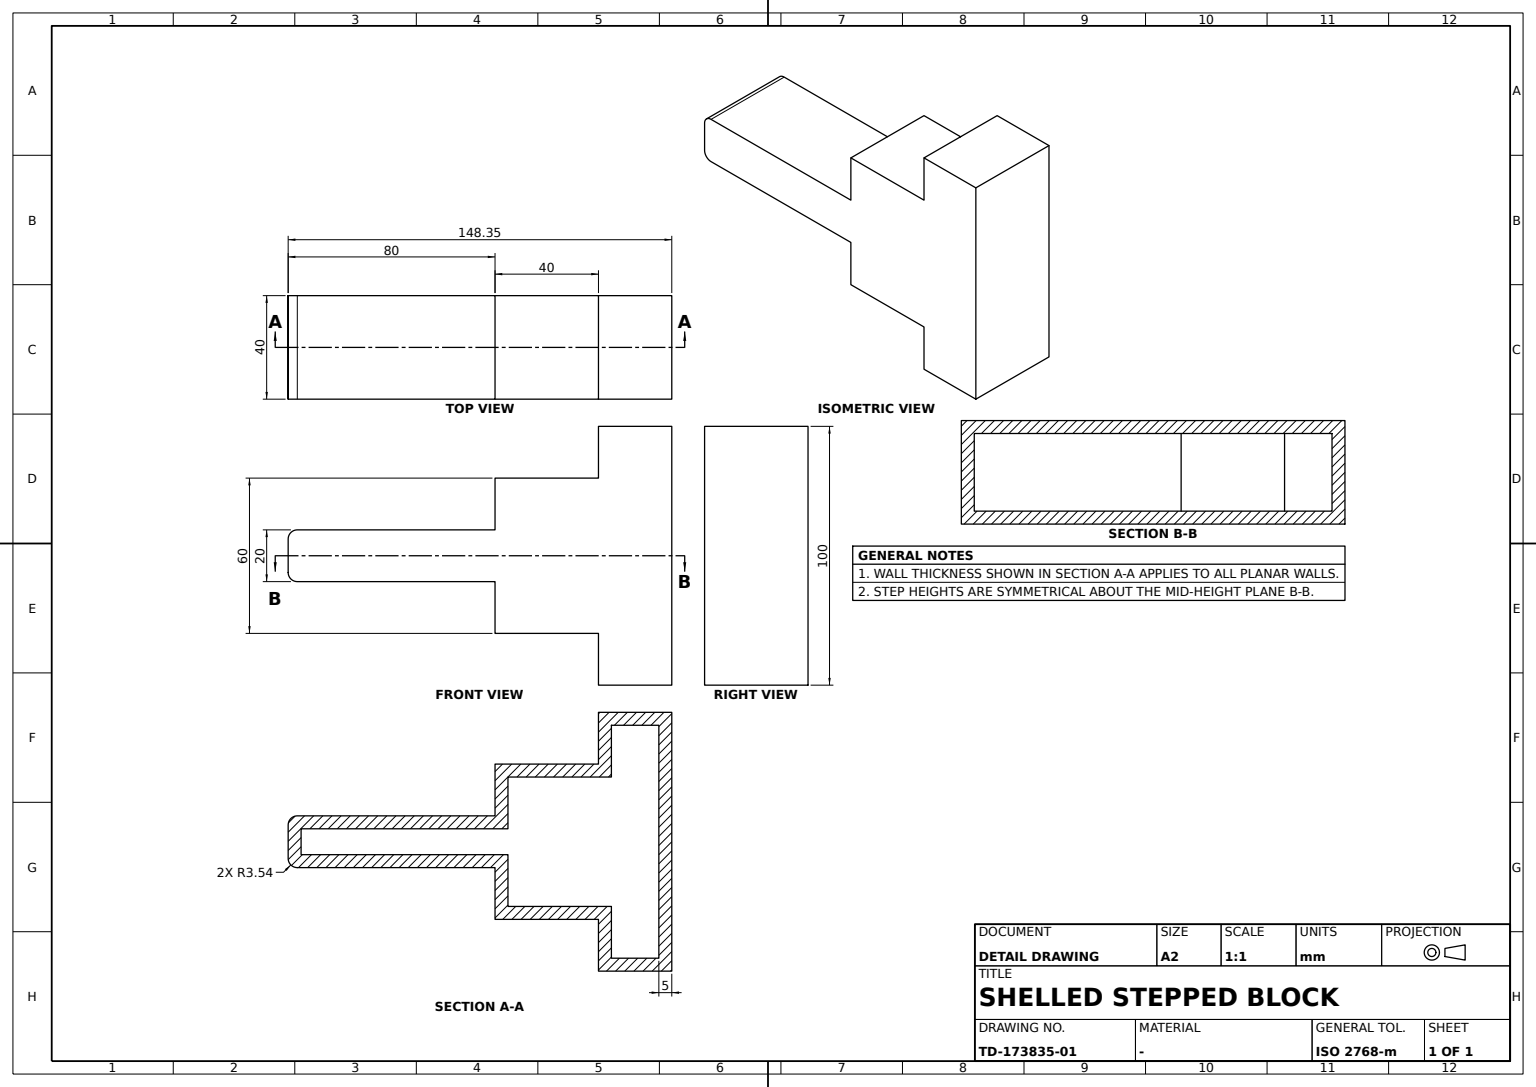
ISO-10303-21;
HEADER;
FILE_DESCRIPTION((''),'2;1');
FILE_NAME('','',(''),(''),'','','');
FILE_SCHEMA(('AUTOMOTIVE_DESIGN'));
ENDSEC;
DATA;
#1=APPLICATION_CONTEXT('');
#2=PRODUCT_CONTEXT('',#1,'mechanical');
#3=PRODUCT('','','',(#2));
#4=PRODUCT_DEFINITION_FORMATION('','',#3);
#5=PRODUCT_DEFINITION_CONTEXT('',#1,'design');
#6=PRODUCT_DEFINITION('','',#4,#5);
#7=PRODUCT_DEFINITION_SHAPE('','',#6);
#8=(LENGTH_UNIT()NAMED_UNIT(*)SI_UNIT(.MILLI.,.METRE.));
#9=(NAMED_UNIT(*)PLANE_ANGLE_UNIT()SI_UNIT($,.RADIAN.));
#10=(NAMED_UNIT(*)SI_UNIT($,.STERADIAN.)SOLID_ANGLE_UNIT());
#11=UNCERTAINTY_MEASURE_WITH_UNIT(LENGTH_MEASURE(0.005),#8,'distance_accuracy_value','');
#12=(GEOMETRIC_REPRESENTATION_CONTEXT(3)GLOBAL_UNCERTAINTY_ASSIGNED_CONTEXT((#11))GLOBAL_UNIT_ASSIGNED_CONTEXT((#8,#9,#10))REPRESENTATION_CONTEXT('',''));
#13=CARTESIAN_POINT('',(-28.352545,30.,-20.));
#14=VERTEX_POINT('',#13);
#15=CARTESIAN_POINT('',(-28.352545,30.,20.));
#16=VERTEX_POINT('',#15);
#17=CARTESIAN_POINT('',(-28.352545,30.,0.));
#18=DIRECTION('',(0.,0.,1.));
#19=VECTOR('',#18,1000.);
#20=LINE('',#17,#19);
#21=EDGE_CURVE('',#14,#16,#20,.T.);
#22=ORIENTED_EDGE('',*,*,#21,.F.);
#23=CARTESIAN_POINT('',(-68.352545,30.,-20.));
#24=VERTEX_POINT('',#23);
#25=CARTESIAN_POINT('',(0.,30.,-20.));
#26=DIRECTION('',(-1.,0.,0.));
#27=VECTOR('',#26,1000.);
#28=LINE('',#25,#27);
#29=EDGE_CURVE('',#14,#24,#28,.T.);
#30=ORIENTED_EDGE('',*,*,#29,.T.);
#31=CARTESIAN_POINT('',(-68.352545,30.,20.));
#32=VERTEX_POINT('',#31);
#33=CARTESIAN_POINT('',(-68.352545,30.,0.));
#34=LINE('',#33,#19);
#35=EDGE_CURVE('',#24,#32,#34,.T.);
#36=ORIENTED_EDGE('',*,*,#35,.T.);
#37=CARTESIAN_POINT('',(0.,30.,20.));
#38=LINE('',#37,#27);
#39=EDGE_CURVE('',#16,#32,#38,.T.);
#40=ORIENTED_EDGE('',*,*,#39,.F.);
#41=EDGE_LOOP('',(#22,#30,#36,#40));
#42=FACE_BOUND('',#41,.T.);
#43=DIRECTION('',(0.,1.,0.));
#44=AXIS2_PLACEMENT_3D('',#17,#43,#26);
#45=PLANE('',#44);
#46=ADVANCED_FACE('',(#42),#45,.T.);
#47=CARTESIAN_POINT('',(-68.352545,10.,-20.));
#48=VERTEX_POINT('',#47);
#49=CARTESIAN_POINT('',(-68.352545,10.,20.));
#50=VERTEX_POINT('',#49);
#51=CARTESIAN_POINT('',(-68.352545,10.,0.));
#52=LINE('',#51,#19);
#53=EDGE_CURVE('',#48,#50,#52,.T.);
#54=ORIENTED_EDGE('',*,*,#53,.T.);
#55=CARTESIAN_POINT('',(-68.352545,0.,20.));
#56=DIRECTION('',(0.,-1.,0.));
#57=VECTOR('',#56,1000.);
#58=LINE('',#55,#57);
#59=EDGE_CURVE('',#32,#50,#58,.T.);
#60=ORIENTED_EDGE('',*,*,#59,.F.);
#61=ORIENTED_EDGE('',*,*,#35,.F.);
#62=CARTESIAN_POINT('',(-68.352545,0.,-20.));
#63=LINE('',#62,#57);
#64=EDGE_CURVE('',#24,#48,#63,.T.);
#65=ORIENTED_EDGE('',*,*,#64,.T.);
#66=EDGE_LOOP('',(#54,#60,#61,#65));
#67=FACE_BOUND('',#66,.T.);
#68=AXIS2_PLACEMENT_3D('',#33,#26,#56);
#69=PLANE('',#68);
#70=ADVANCED_FACE('',(#67),#69,.T.);
#71=CARTESIAN_POINT('',(-28.352545,-30.,-20.));
#72=VERTEX_POINT('',#71);
#73=CARTESIAN_POINT('',(-28.352545,-30.,20.));
#74=VERTEX_POINT('',#73);
#75=CARTESIAN_POINT('',(-28.352545,-30.,0.));
#76=LINE('',#75,#19);
#77=EDGE_CURVE('',#72,#74,#76,.T.);
#78=ORIENTED_EDGE('',*,*,#77,.T.);
#79=CARTESIAN_POINT('',(-68.352545,-30.,20.));
#80=VERTEX_POINT('',#79);
#81=CARTESIAN_POINT('',(0.,-30.,20.));
#82=DIRECTION('',(1.,0.,0.));
#83=VECTOR('',#82,1000.);
#84=LINE('',#81,#83);
#85=EDGE_CURVE('',#80,#74,#84,.T.);
#86=ORIENTED_EDGE('',*,*,#85,.F.);
#87=CARTESIAN_POINT('',(-68.352545,-30.,-20.));
#88=VERTEX_POINT('',#87);
#89=CARTESIAN_POINT('',(-68.352545,-30.,0.));
#90=LINE('',#89,#19);
#91=EDGE_CURVE('',#88,#80,#90,.T.);
#92=ORIENTED_EDGE('',*,*,#91,.F.);
#93=CARTESIAN_POINT('',(0.,-30.,-20.));
#94=LINE('',#93,#83);
#95=EDGE_CURVE('',#88,#72,#94,.T.);
#96=ORIENTED_EDGE('',*,*,#95,.T.);
#97=EDGE_LOOP('',(#78,#86,#92,#96));
#98=FACE_BOUND('',#97,.T.);
#99=AXIS2_PLACEMENT_3D('',#89,#56,#82);
#100=PLANE('',#99);
#101=ADVANCED_FACE('',(#98),#100,.T.);
#102=CARTESIAN_POINT('',(0.,-50.,20.));
#103=VERTEX_POINT('',#102);
#104=CARTESIAN_POINT('',(-28.352545,-50.,20.));
#105=VERTEX_POINT('',#104);
#106=LINE('',#102,#27);
#107=EDGE_CURVE('',#103,#105,#106,.T.);
#108=ORIENTED_EDGE('',*,*,#107,.F.);
#109=CARTESIAN_POINT('',(0.,50.,20.));
#110=VERTEX_POINT('',#109);
#111=CARTESIAN_POINT('',(0.,0.,20.));
#112=VECTOR('',#43,1000.);
#113=LINE('',#111,#112);
#114=EDGE_CURVE('',#103,#110,#113,.T.);
#115=ORIENTED_EDGE('',*,*,#114,.T.);
#116=CARTESIAN_POINT('',(-28.352545,50.,20.));
#117=VERTEX_POINT('',#116);
#118=LINE('',#109,#27);
#119=EDGE_CURVE('',#110,#117,#118,.T.);
#120=ORIENTED_EDGE('',*,*,#119,.T.);
#121=CARTESIAN_POINT('',(-28.352545,0.,20.));
#122=LINE('',#121,#57);
#123=EDGE_CURVE('',#117,#16,#122,.T.);
#124=ORIENTED_EDGE('',*,*,#123,.T.);
#125=ORIENTED_EDGE('',*,*,#39,.T.);
#126=ORIENTED_EDGE('',*,*,#59,.T.);
#127=CARTESIAN_POINT('',(-144.817011,10.,20.));
#128=VERTEX_POINT('',#127);
#129=CARTESIAN_POINT('',(0.,10.,20.));
#130=LINE('',#129,#27);
#131=EDGE_CURVE('',#50,#128,#130,.T.);
#132=ORIENTED_EDGE('',*,*,#131,.T.);
#133=CARTESIAN_POINT('',(-148.352545,6.464466,20.));
#134=VERTEX_POINT('',#133);
#135=CARTESIAN_POINT('',(-144.817011,6.464466,20.));
#136=AXIS2_PLACEMENT_3D('',#135,#18,#82);
#137=CIRCLE('',#136,3.535534);
#138=EDGE_CURVE('',#128,#134,#137,.T.);
#139=ORIENTED_EDGE('',*,*,#138,.T.);
#140=CARTESIAN_POINT('',(-148.352545,-6.464466,20.));
#141=VERTEX_POINT('',#140);
#142=CARTESIAN_POINT('',(-148.352545,0.,20.));
#143=LINE('',#142,#57);
#144=EDGE_CURVE('',#134,#141,#143,.T.);
#145=ORIENTED_EDGE('',*,*,#144,.T.);
#146=CARTESIAN_POINT('',(-144.817011,-10.,20.));
#147=VERTEX_POINT('',#146);
#148=CARTESIAN_POINT('',(-144.817011,-6.464466,20.));
#149=AXIS2_PLACEMENT_3D('',#148,#18,#82);
#150=CIRCLE('',#149,3.535534);
#151=EDGE_CURVE('',#141,#147,#150,.T.);
#152=ORIENTED_EDGE('',*,*,#151,.T.);
#153=CARTESIAN_POINT('',(-68.352545,-10.,20.));
#154=VERTEX_POINT('',#153);
#155=CARTESIAN_POINT('',(0.,-10.,20.));
#156=LINE('',#155,#83);
#157=EDGE_CURVE('',#147,#154,#156,.T.);
#158=ORIENTED_EDGE('',*,*,#157,.T.);
#159=EDGE_CURVE('',#154,#80,#58,.T.);
#160=ORIENTED_EDGE('',*,*,#159,.T.);
#161=ORIENTED_EDGE('',*,*,#85,.T.);
#162=EDGE_CURVE('',#74,#105,#122,.T.);
#163=ORIENTED_EDGE('',*,*,#162,.T.);
#164=EDGE_LOOP('',(#108,#115,#120,#124,#125,#126,#132,#139,#145,#152,#158,#160,#161,#163));
#165=FACE_BOUND('',#164,.T.);
#166=AXIS2_PLACEMENT_3D('',#111,#18,#82);
#167=PLANE('',#166);
#168=ADVANCED_FACE('',(#165),#167,.T.);
#169=CARTESIAN_POINT('',(-28.352545,-50.,-20.));
#170=VERTEX_POINT('',#169);
#171=CARTESIAN_POINT('',(-28.352545,0.,-20.));
#172=LINE('',#171,#57);
#173=EDGE_CURVE('',#72,#170,#172,.T.);
#174=ORIENTED_EDGE('',*,*,#173,.T.);
#175=CARTESIAN_POINT('',(-28.352545,-50.,0.));
#176=LINE('',#175,#19);
#177=EDGE_CURVE('',#170,#105,#176,.T.);
#178=ORIENTED_EDGE('',*,*,#177,.T.);
#179=ORIENTED_EDGE('',*,*,#162,.F.);
#180=ORIENTED_EDGE('',*,*,#77,.F.);
#181=EDGE_LOOP('',(#174,#178,#179,#180));
#182=FACE_BOUND('',#181,.T.);
#183=CARTESIAN_POINT('',(-28.352545,50.,0.));
#184=AXIS2_PLACEMENT_3D('',#183,#26,#56);
#185=PLANE('',#184);
#186=ADVANCED_FACE('',(#182),#185,.T.);
#187=ORIENTED_EDGE('',*,*,#29,.F.);
#188=CARTESIAN_POINT('',(-28.352545,50.,-20.));
#189=VERTEX_POINT('',#188);
#190=EDGE_CURVE('',#189,#14,#172,.T.);
#191=ORIENTED_EDGE('',*,*,#190,.F.);
#192=CARTESIAN_POINT('',(0.,50.,-20.));
#193=VERTEX_POINT('',#192);
#194=LINE('',#192,#27);
#195=EDGE_CURVE('',#193,#189,#194,.T.);
#196=ORIENTED_EDGE('',*,*,#195,.F.);
#197=CARTESIAN_POINT('',(0.,-50.,-20.));
#198=VERTEX_POINT('',#197);
#199=CARTESIAN_POINT('',(0.,0.,-20.));
#200=LINE('',#199,#112);
#201=EDGE_CURVE('',#198,#193,#200,.T.);
#202=ORIENTED_EDGE('',*,*,#201,.F.);
#203=LINE('',#197,#27);
#204=EDGE_CURVE('',#198,#170,#203,.T.);
#205=ORIENTED_EDGE('',*,*,#204,.T.);
#206=ORIENTED_EDGE('',*,*,#173,.F.);
#207=ORIENTED_EDGE('',*,*,#95,.F.);
#208=CARTESIAN_POINT('',(-68.352545,-10.,-20.));
#209=VERTEX_POINT('',#208);
#210=EDGE_CURVE('',#209,#88,#63,.T.);
#211=ORIENTED_EDGE('',*,*,#210,.F.);
#212=CARTESIAN_POINT('',(-144.817011,-10.,-20.));
#213=VERTEX_POINT('',#212);
#214=CARTESIAN_POINT('',(0.,-10.,-20.));
#215=LINE('',#214,#83);
#216=EDGE_CURVE('',#213,#209,#215,.T.);
#217=ORIENTED_EDGE('',*,*,#216,.F.);
#218=CARTESIAN_POINT('',(-148.352545,-6.464466,-20.));
#219=VERTEX_POINT('',#218);
#220=CARTESIAN_POINT('',(-144.817011,-6.464466,-20.));
#221=AXIS2_PLACEMENT_3D('',#220,#18,#82);
#222=CIRCLE('',#221,3.535534);
#223=EDGE_CURVE('',#219,#213,#222,.T.);
#224=ORIENTED_EDGE('',*,*,#223,.F.);
#225=CARTESIAN_POINT('',(-148.352545,6.464466,-20.));
#226=VERTEX_POINT('',#225);
#227=CARTESIAN_POINT('',(-148.352545,0.,-20.));
#228=LINE('',#227,#57);
#229=EDGE_CURVE('',#226,#219,#228,.T.);
#230=ORIENTED_EDGE('',*,*,#229,.F.);
#231=CARTESIAN_POINT('',(-144.817011,10.,-20.));
#232=VERTEX_POINT('',#231);
#233=CARTESIAN_POINT('',(-144.817011,6.464466,-20.));
#234=AXIS2_PLACEMENT_3D('',#233,#18,#82);
#235=CIRCLE('',#234,3.535534);
#236=EDGE_CURVE('',#232,#226,#235,.T.);
#237=ORIENTED_EDGE('',*,*,#236,.F.);
#238=CARTESIAN_POINT('',(0.,10.,-20.));
#239=LINE('',#238,#27);
#240=EDGE_CURVE('',#48,#232,#239,.T.);
#241=ORIENTED_EDGE('',*,*,#240,.F.);
#242=ORIENTED_EDGE('',*,*,#64,.F.);
#243=EDGE_LOOP('',(#187,#191,#196,#202,#205,#206,#207,#211,#217,#224,#230,#237,#241,#242));
#244=FACE_BOUND('',#243,.T.);
#245=AXIS2_PLACEMENT_3D('',#199,#18,#82);
#246=PLANE('',#245);
#247=ADVANCED_FACE('',(#244),#246,.F.);
#248=ORIENTED_EDGE('',*,*,#144,.F.);
#249=CARTESIAN_POINT('',(-148.352545,6.464466,0.));
#250=DIRECTION('',(0.,0.,-1.));
#251=VECTOR('',#250,1000.);
#252=LINE('',#249,#251);
#253=EDGE_CURVE('',#134,#226,#252,.T.);
#254=ORIENTED_EDGE('',*,*,#253,.T.);
#255=ORIENTED_EDGE('',*,*,#229,.T.);
#256=CARTESIAN_POINT('',(-148.352545,-6.464466,0.));
#257=LINE('',#256,#251);
#258=EDGE_CURVE('',#141,#219,#257,.T.);
#259=ORIENTED_EDGE('',*,*,#258,.F.);
#260=EDGE_LOOP('',(#248,#254,#255,#259));
#261=FACE_BOUND('',#260,.T.);
#262=CARTESIAN_POINT('',(-148.352545,10.,0.));
#263=AXIS2_PLACEMENT_3D('',#262,#26,#56);
#264=PLANE('',#263);
#265=ADVANCED_FACE('',(#261),#264,.T.);
#266=ORIENTED_EDGE('',*,*,#151,.F.);
#267=ORIENTED_EDGE('',*,*,#258,.T.);
#268=ORIENTED_EDGE('',*,*,#223,.T.);
#269=CARTESIAN_POINT('',(-144.817011,-10.,0.));
#270=LINE('',#269,#251);
#271=EDGE_CURVE('',#147,#213,#270,.T.);
#272=ORIENTED_EDGE('',*,*,#271,.F.);
#273=EDGE_LOOP('',(#266,#267,#268,#272));
#274=FACE_BOUND('',#273,.T.);
#275=CARTESIAN_POINT('',(-144.817011,-6.464466,0.));
#276=AXIS2_PLACEMENT_3D('',#275,#250,#56);
#277=CYLINDRICAL_SURFACE('',#276,3.535534);
#278=ADVANCED_FACE('',(#274),#277,.T.);
#279=LINE('',#183,#19);
#280=EDGE_CURVE('',#189,#117,#279,.T.);
#281=ORIENTED_EDGE('',*,*,#280,.F.);
#282=ORIENTED_EDGE('',*,*,#190,.T.);
#283=ORIENTED_EDGE('',*,*,#21,.T.);
#284=ORIENTED_EDGE('',*,*,#123,.F.);
#285=EDGE_LOOP('',(#281,#282,#283,#284));
#286=FACE_BOUND('',#285,.T.);
#287=ADVANCED_FACE('',(#286),#185,.T.);
#288=ORIENTED_EDGE('',*,*,#107,.T.);
#289=ORIENTED_EDGE('',*,*,#177,.F.);
#290=ORIENTED_EDGE('',*,*,#204,.F.);
#291=CARTESIAN_POINT('',(0.,-50.,0.));
#292=LINE('',#291,#19);
#293=EDGE_CURVE('',#198,#103,#292,.T.);
#294=ORIENTED_EDGE('',*,*,#293,.T.);
#295=EDGE_LOOP('',(#288,#289,#290,#294));
#296=FACE_BOUND('',#295,.T.);
#297=AXIS2_PLACEMENT_3D('',#291,#43,#26);
#298=PLANE('',#297);
#299=ADVANCED_FACE('',(#296),#298,.F.);
#300=ORIENTED_EDGE('',*,*,#53,.F.);
#301=ORIENTED_EDGE('',*,*,#240,.T.);
#302=CARTESIAN_POINT('',(-144.817011,10.,0.));
#303=LINE('',#302,#251);
#304=EDGE_CURVE('',#128,#232,#303,.T.);
#305=ORIENTED_EDGE('',*,*,#304,.F.);
#306=ORIENTED_EDGE('',*,*,#131,.F.);
#307=EDGE_LOOP('',(#300,#301,#305,#306));
#308=FACE_BOUND('',#307,.T.);
#309=AXIS2_PLACEMENT_3D('',#51,#43,#26);
#310=PLANE('',#309);
#311=ADVANCED_FACE('',(#308),#310,.T.);
#312=CARTESIAN_POINT('',(0.,50.,0.));
#313=LINE('',#312,#19);
#314=EDGE_CURVE('',#193,#110,#313,.T.);
#315=ORIENTED_EDGE('',*,*,#314,.F.);
#316=ORIENTED_EDGE('',*,*,#195,.T.);
#317=ORIENTED_EDGE('',*,*,#280,.T.);
#318=ORIENTED_EDGE('',*,*,#119,.F.);
#319=EDGE_LOOP('',(#315,#316,#317,#318));
#320=FACE_BOUND('',#319,.T.);
#321=AXIS2_PLACEMENT_3D('',#312,#43,#26);
#322=PLANE('',#321);
#323=ADVANCED_FACE('',(#320),#322,.T.);
#324=ORIENTED_EDGE('',*,*,#159,.F.);
#325=CARTESIAN_POINT('',(-68.352545,-10.,0.));
#326=LINE('',#325,#19);
#327=EDGE_CURVE('',#209,#154,#326,.T.);
#328=ORIENTED_EDGE('',*,*,#327,.F.);
#329=ORIENTED_EDGE('',*,*,#210,.T.);
#330=ORIENTED_EDGE('',*,*,#91,.T.);
#331=EDGE_LOOP('',(#324,#328,#329,#330));
#332=FACE_BOUND('',#331,.T.);
#333=ADVANCED_FACE('',(#332),#69,.T.);
#334=ORIENTED_EDGE('',*,*,#236,.T.);
#335=ORIENTED_EDGE('',*,*,#253,.F.);
#336=ORIENTED_EDGE('',*,*,#138,.F.);
#337=ORIENTED_EDGE('',*,*,#304,.T.);
#338=EDGE_LOOP('',(#334,#335,#336,#337));
#339=FACE_BOUND('',#338,.T.);
#340=CARTESIAN_POINT('',(-144.817011,6.464466,0.));
#341=AXIS2_PLACEMENT_3D('',#340,#250,#26);
#342=CYLINDRICAL_SURFACE('',#341,3.535534);
#343=ADVANCED_FACE('',(#339),#342,.T.);
#344=ORIENTED_EDGE('',*,*,#114,.F.);
#345=ORIENTED_EDGE('',*,*,#293,.F.);
#346=ORIENTED_EDGE('',*,*,#201,.T.);
#347=ORIENTED_EDGE('',*,*,#314,.T.);
#348=EDGE_LOOP('',(#344,#345,#346,#347));
#349=FACE_BOUND('',#348,.T.);
#350=AXIS2_PLACEMENT_3D('',#291,#82,#43);
#351=PLANE('',#350);
#352=ADVANCED_FACE('',(#349),#351,.T.);
#353=ORIENTED_EDGE('',*,*,#157,.F.);
#354=ORIENTED_EDGE('',*,*,#271,.T.);
#355=ORIENTED_EDGE('',*,*,#216,.T.);
#356=ORIENTED_EDGE('',*,*,#327,.T.);
#357=EDGE_LOOP('',(#353,#354,#355,#356));
#358=FACE_BOUND('',#357,.T.);
#359=CARTESIAN_POINT('',(-148.352545,-10.,0.));
#360=AXIS2_PLACEMENT_3D('',#359,#56,#82);
#361=PLANE('',#360);
#362=ADVANCED_FACE('',(#358),#361,.T.);
#363=CLOSED_SHELL('',(#46,#70,#101,#168,#186,#247,#265,#278,#287,#299,#311,#323,#333,#343,#352,#362));
#364=CARTESIAN_POINT('',(-23.352545,-45.,15.));
#365=VERTEX_POINT('',#364);
#366=CARTESIAN_POINT('',(-5.,-45.,15.));
#367=VERTEX_POINT('',#366);
#368=CARTESIAN_POINT('',(0.,-45.,15.));
#369=LINE('',#368,#83);
#370=EDGE_CURVE('',#365,#367,#369,.T.);
#371=ORIENTED_EDGE('',*,*,#370,.F.);
#372=CARTESIAN_POINT('',(-23.352545,-25.,15.));
#373=VERTEX_POINT('',#372);
#374=CARTESIAN_POINT('',(-23.352545,50.,15.));
#375=LINE('',#374,#112);
#376=EDGE_CURVE('',#365,#373,#375,.T.);
#377=ORIENTED_EDGE('',*,*,#376,.T.);
#378=CARTESIAN_POINT('',(-63.352545,-25.,15.));
#379=VERTEX_POINT('',#378);
#380=CARTESIAN_POINT('',(0.,-25.,15.));
#381=LINE('',#380,#83);
#382=EDGE_CURVE('',#379,#373,#381,.T.);
#383=ORIENTED_EDGE('',*,*,#382,.F.);
#384=CARTESIAN_POINT('',(-63.352545,-5.,15.));
#385=VERTEX_POINT('',#384);
#386=CARTESIAN_POINT('',(-63.352545,30.,15.));
#387=LINE('',#386,#112);
#388=EDGE_CURVE('',#379,#385,#387,.T.);
#389=ORIENTED_EDGE('',*,*,#388,.T.);
#390=CARTESIAN_POINT('',(-143.352545,-5.,15.));
#391=VERTEX_POINT('',#390);
#392=CARTESIAN_POINT('',(-148.352545,-5.,15.));
#393=LINE('',#392,#27);
#394=EDGE_CURVE('',#385,#391,#393,.T.);
#395=ORIENTED_EDGE('',*,*,#394,.T.);
#396=CARTESIAN_POINT('',(-143.352545,5.,15.));
#397=VERTEX_POINT('',#396);
#398=CARTESIAN_POINT('',(-143.352545,10.,15.));
#399=LINE('',#398,#112);
#400=EDGE_CURVE('',#391,#397,#399,.T.);
#401=ORIENTED_EDGE('',*,*,#400,.T.);
#402=CARTESIAN_POINT('',(-63.352545,5.,15.));
#403=VERTEX_POINT('',#402);
#404=CARTESIAN_POINT('',(-68.352545,5.,15.));
#405=LINE('',#404,#83);
#406=EDGE_CURVE('',#397,#403,#405,.T.);
#407=ORIENTED_EDGE('',*,*,#406,.T.);
#408=CARTESIAN_POINT('',(-63.352545,25.,15.));
#409=VERTEX_POINT('',#408);
#410=EDGE_CURVE('',#403,#409,#387,.T.);
#411=ORIENTED_EDGE('',*,*,#410,.T.);
#412=CARTESIAN_POINT('',(-23.352545,25.,15.));
#413=VERTEX_POINT('',#412);
#414=CARTESIAN_POINT('',(0.,25.,15.));
#415=LINE('',#414,#27);
#416=EDGE_CURVE('',#413,#409,#415,.T.);
#417=ORIENTED_EDGE('',*,*,#416,.F.);
#418=CARTESIAN_POINT('',(-23.352545,45.,15.));
#419=VERTEX_POINT('',#418);
#420=EDGE_CURVE('',#413,#419,#375,.T.);
#421=ORIENTED_EDGE('',*,*,#420,.T.);
#422=CARTESIAN_POINT('',(-5.,45.,15.));
#423=VERTEX_POINT('',#422);
#424=CARTESIAN_POINT('',(0.,45.,15.));
#425=LINE('',#424,#27);
#426=EDGE_CURVE('',#423,#419,#425,.T.);
#427=ORIENTED_EDGE('',*,*,#426,.F.);
#428=CARTESIAN_POINT('',(-5.,-50.,15.));
#429=LINE('',#428,#57);
#430=EDGE_CURVE('',#423,#367,#429,.T.);
#431=ORIENTED_EDGE('',*,*,#430,.T.);
#432=EDGE_LOOP('',(#371,#377,#383,#389,#395,#401,#407,#411,#417,#421,#427,#431));
#433=FACE_BOUND('',#432,.T.);
#434=CARTESIAN_POINT('',(0.,0.,15.));
#435=AXIS2_PLACEMENT_3D('',#434,#18,#82);
#436=PLANE('',#435);
#437=ADVANCED_FACE('',(#433),#436,.F.);
#438=ORIENTED_EDGE('',*,*,#400,.F.);
#439=CARTESIAN_POINT('',(-143.352545,-5.,-15.));
#440=VERTEX_POINT('',#439);
#441=CARTESIAN_POINT('',(-143.352545,-5.,0.));
#442=LINE('',#441,#251);
#443=EDGE_CURVE('',#391,#440,#442,.T.);
#444=ORIENTED_EDGE('',*,*,#443,.T.);
#445=CARTESIAN_POINT('',(-143.352545,5.,-15.));
#446=VERTEX_POINT('',#445);
#447=CARTESIAN_POINT('',(-143.352545,10.,-15.));
#448=LINE('',#447,#112);
#449=EDGE_CURVE('',#440,#446,#448,.T.);
#450=ORIENTED_EDGE('',*,*,#449,.T.);
#451=CARTESIAN_POINT('',(-143.352545,5.,0.));
#452=LINE('',#451,#19);
#453=EDGE_CURVE('',#446,#397,#452,.T.);
#454=ORIENTED_EDGE('',*,*,#453,.T.);
#455=EDGE_LOOP('',(#438,#444,#450,#454));
#456=FACE_BOUND('',#455,.T.);
#457=CARTESIAN_POINT('',(-143.352545,10.,0.));
#458=AXIS2_PLACEMENT_3D('',#457,#26,#56);
#459=PLANE('',#458);
#460=ADVANCED_FACE('',(#456),#459,.F.);
#461=ORIENTED_EDGE('',*,*,#443,.F.);
#462=ORIENTED_EDGE('',*,*,#394,.F.);
#463=CARTESIAN_POINT('',(-63.352545,-5.,-15.));
#464=VERTEX_POINT('',#463);
#465=CARTESIAN_POINT('',(-63.352545,-5.,0.));
#466=LINE('',#465,#19);
#467=EDGE_CURVE('',#464,#385,#466,.T.);
#468=ORIENTED_EDGE('',*,*,#467,.F.);
#469=CARTESIAN_POINT('',(-148.352545,-5.,-15.));
#470=LINE('',#469,#27);
#471=EDGE_CURVE('',#464,#440,#470,.T.);
#472=ORIENTED_EDGE('',*,*,#471,.T.);
#473=EDGE_LOOP('',(#461,#462,#468,#472));
#474=FACE_BOUND('',#473,.T.);
#475=CARTESIAN_POINT('',(-148.352545,-5.,0.));
#476=AXIS2_PLACEMENT_3D('',#475,#56,#82);
#477=PLANE('',#476);
#478=ADVANCED_FACE('',(#474),#477,.F.);
#479=ORIENTED_EDGE('',*,*,#467,.T.);
#480=ORIENTED_EDGE('',*,*,#388,.F.);
#481=CARTESIAN_POINT('',(-63.352545,-25.,-15.));
#482=VERTEX_POINT('',#481);
#483=CARTESIAN_POINT('',(-63.352545,-25.,0.));
#484=LINE('',#483,#19);
#485=EDGE_CURVE('',#482,#379,#484,.T.);
#486=ORIENTED_EDGE('',*,*,#485,.F.);
#487=CARTESIAN_POINT('',(-63.352545,30.,-15.));
#488=LINE('',#487,#112);
#489=EDGE_CURVE('',#482,#464,#488,.T.);
#490=ORIENTED_EDGE('',*,*,#489,.T.);
#491=EDGE_LOOP('',(#479,#480,#486,#490));
#492=FACE_BOUND('',#491,.T.);
#493=CARTESIAN_POINT('',(-63.352545,30.,0.));
#494=AXIS2_PLACEMENT_3D('',#493,#26,#56);
#495=PLANE('',#494);
#496=ADVANCED_FACE('',(#492),#495,.F.);
#497=ORIENTED_EDGE('',*,*,#485,.T.);
#498=ORIENTED_EDGE('',*,*,#382,.T.);
#499=CARTESIAN_POINT('',(-23.352545,-25.,-15.));
#500=VERTEX_POINT('',#499);
#501=CARTESIAN_POINT('',(-23.352545,-25.,0.));
#502=LINE('',#501,#19);
#503=EDGE_CURVE('',#500,#373,#502,.T.);
#504=ORIENTED_EDGE('',*,*,#503,.F.);
#505=CARTESIAN_POINT('',(0.,-25.,-15.));
#506=LINE('',#505,#83);
#507=EDGE_CURVE('',#482,#500,#506,.T.);
#508=ORIENTED_EDGE('',*,*,#507,.F.);
#509=EDGE_LOOP('',(#497,#498,#504,#508));
#510=FACE_BOUND('',#509,.T.);
#511=CARTESIAN_POINT('',(-68.352545,-25.,0.));
#512=AXIS2_PLACEMENT_3D('',#511,#56,#82);
#513=PLANE('',#512);
#514=ADVANCED_FACE('',(#510),#513,.F.);
#515=ORIENTED_EDGE('',*,*,#406,.F.);
#516=ORIENTED_EDGE('',*,*,#453,.F.);
#517=CARTESIAN_POINT('',(-63.352545,5.,-15.));
#518=VERTEX_POINT('',#517);
#519=CARTESIAN_POINT('',(-68.352545,5.,-15.));
#520=LINE('',#519,#83);
#521=EDGE_CURVE('',#446,#518,#520,.T.);
#522=ORIENTED_EDGE('',*,*,#521,.T.);
#523=CARTESIAN_POINT('',(-63.352545,5.,0.));
#524=LINE('',#523,#19);
#525=EDGE_CURVE('',#518,#403,#524,.T.);
#526=ORIENTED_EDGE('',*,*,#525,.T.);
#527=EDGE_LOOP('',(#515,#516,#522,#526));
#528=FACE_BOUND('',#527,.T.);
#529=CARTESIAN_POINT('',(-68.352545,5.,0.));
#530=AXIS2_PLACEMENT_3D('',#529,#43,#26);
#531=PLANE('',#530);
#532=ADVANCED_FACE('',(#528),#531,.F.);
#533=ORIENTED_EDGE('',*,*,#416,.T.);
#534=CARTESIAN_POINT('',(-63.352545,25.,-15.));
#535=VERTEX_POINT('',#534);
#536=CARTESIAN_POINT('',(-63.352545,25.,0.));
#537=LINE('',#536,#19);
#538=EDGE_CURVE('',#535,#409,#537,.T.);
#539=ORIENTED_EDGE('',*,*,#538,.F.);
#540=CARTESIAN_POINT('',(-23.352545,25.,-15.));
#541=VERTEX_POINT('',#540);
#542=CARTESIAN_POINT('',(0.,25.,-15.));
#543=LINE('',#542,#27);
#544=EDGE_CURVE('',#541,#535,#543,.T.);
#545=ORIENTED_EDGE('',*,*,#544,.F.);
#546=CARTESIAN_POINT('',(-23.352545,25.,0.));
#547=LINE('',#546,#19);
#548=EDGE_CURVE('',#541,#413,#547,.T.);
#549=ORIENTED_EDGE('',*,*,#548,.T.);
#550=EDGE_LOOP('',(#533,#539,#545,#549));
#551=FACE_BOUND('',#550,.T.);
#552=CARTESIAN_POINT('',(-28.352545,25.,0.));
#553=AXIS2_PLACEMENT_3D('',#552,#43,#26);
#554=PLANE('',#553);
#555=ADVANCED_FACE('',(#551),#554,.F.);
#556=CARTESIAN_POINT('',(-23.352545,-45.,-15.));
#557=VERTEX_POINT('',#556);
#558=CARTESIAN_POINT('',(-23.352545,-45.,0.));
#559=LINE('',#558,#19);
#560=EDGE_CURVE('',#557,#365,#559,.T.);
#561=ORIENTED_EDGE('',*,*,#560,.F.);
#562=CARTESIAN_POINT('',(-23.352545,50.,-15.));
#563=LINE('',#562,#112);
#564=EDGE_CURVE('',#557,#500,#563,.T.);
#565=ORIENTED_EDGE('',*,*,#564,.T.);
#566=ORIENTED_EDGE('',*,*,#503,.T.);
#567=ORIENTED_EDGE('',*,*,#376,.F.);
#568=EDGE_LOOP('',(#561,#565,#566,#567));
#569=FACE_BOUND('',#568,.T.);
#570=CARTESIAN_POINT('',(-23.352545,50.,0.));
#571=AXIS2_PLACEMENT_3D('',#570,#26,#56);
#572=PLANE('',#571);
#573=ADVANCED_FACE('',(#569),#572,.F.);
#574=ORIENTED_EDGE('',*,*,#426,.T.);
#575=CARTESIAN_POINT('',(-23.352545,45.,-15.));
#576=VERTEX_POINT('',#575);
#577=CARTESIAN_POINT('',(-23.352545,45.,0.));
#578=LINE('',#577,#19);
#579=EDGE_CURVE('',#576,#419,#578,.T.);
#580=ORIENTED_EDGE('',*,*,#579,.F.);
#581=CARTESIAN_POINT('',(-5.,45.,-15.));
#582=VERTEX_POINT('',#581);
#583=CARTESIAN_POINT('',(0.,45.,-15.));
#584=LINE('',#583,#27);
#585=EDGE_CURVE('',#582,#576,#584,.T.);
#586=ORIENTED_EDGE('',*,*,#585,.F.);
#587=CARTESIAN_POINT('',(-5.,45.,0.));
#588=LINE('',#587,#19);
#589=EDGE_CURVE('',#582,#423,#588,.T.);
#590=ORIENTED_EDGE('',*,*,#589,.T.);
#591=EDGE_LOOP('',(#574,#580,#586,#590));
#592=FACE_BOUND('',#591,.T.);
#593=CARTESIAN_POINT('',(0.,45.,0.));
#594=AXIS2_PLACEMENT_3D('',#593,#43,#26);
#595=PLANE('',#594);
#596=ADVANCED_FACE('',(#592),#595,.F.);
#597=ORIENTED_EDGE('',*,*,#589,.F.);
#598=CARTESIAN_POINT('',(-5.,-45.,-15.));
#599=VERTEX_POINT('',#598);
#600=CARTESIAN_POINT('',(-5.,-50.,-15.));
#601=LINE('',#600,#57);
#602=EDGE_CURVE('',#582,#599,#601,.T.);
#603=ORIENTED_EDGE('',*,*,#602,.T.);
#604=CARTESIAN_POINT('',(-5.,-45.,0.));
#605=LINE('',#604,#19);
#606=EDGE_CURVE('',#599,#367,#605,.T.);
#607=ORIENTED_EDGE('',*,*,#606,.T.);
#608=ORIENTED_EDGE('',*,*,#430,.F.);
#609=EDGE_LOOP('',(#597,#603,#607,#608));
#610=FACE_BOUND('',#609,.T.);
#611=CARTESIAN_POINT('',(-5.,-50.,0.));
#612=AXIS2_PLACEMENT_3D('',#611,#82,#43);
#613=PLANE('',#612);
#614=ADVANCED_FACE('',(#610),#613,.F.);
#615=EDGE_CURVE('',#518,#535,#488,.T.);
#616=ORIENTED_EDGE('',*,*,#615,.T.);
#617=ORIENTED_EDGE('',*,*,#538,.T.);
#618=ORIENTED_EDGE('',*,*,#410,.F.);
#619=ORIENTED_EDGE('',*,*,#525,.F.);
#620=EDGE_LOOP('',(#616,#617,#618,#619));
#621=FACE_BOUND('',#620,.T.);
#622=ADVANCED_FACE('',(#621),#495,.F.);
#623=ORIENTED_EDGE('',*,*,#560,.T.);
#624=ORIENTED_EDGE('',*,*,#370,.T.);
#625=ORIENTED_EDGE('',*,*,#606,.F.);
#626=CARTESIAN_POINT('',(0.,-45.,-15.));
#627=LINE('',#626,#83);
#628=EDGE_CURVE('',#557,#599,#627,.T.);
#629=ORIENTED_EDGE('',*,*,#628,.F.);
#630=EDGE_LOOP('',(#623,#624,#625,#629));
#631=FACE_BOUND('',#630,.T.);
#632=CARTESIAN_POINT('',(0.,-45.,0.));
#633=AXIS2_PLACEMENT_3D('',#632,#43,#26);
#634=PLANE('',#633);
#635=ADVANCED_FACE('',(#631),#634,.T.);
#636=EDGE_CURVE('',#541,#576,#563,.T.);
#637=ORIENTED_EDGE('',*,*,#636,.T.);
#638=ORIENTED_EDGE('',*,*,#579,.T.);
#639=ORIENTED_EDGE('',*,*,#420,.F.);
#640=ORIENTED_EDGE('',*,*,#548,.F.);
#641=EDGE_LOOP('',(#637,#638,#639,#640));
#642=FACE_BOUND('',#641,.T.);
#643=ADVANCED_FACE('',(#642),#572,.F.);
#644=ORIENTED_EDGE('',*,*,#602,.F.);
#645=ORIENTED_EDGE('',*,*,#585,.T.);
#646=ORIENTED_EDGE('',*,*,#636,.F.);
#647=ORIENTED_EDGE('',*,*,#544,.T.);
#648=ORIENTED_EDGE('',*,*,#615,.F.);
#649=ORIENTED_EDGE('',*,*,#521,.F.);
#650=ORIENTED_EDGE('',*,*,#449,.F.);
#651=ORIENTED_EDGE('',*,*,#471,.F.);
#652=ORIENTED_EDGE('',*,*,#489,.F.);
#653=ORIENTED_EDGE('',*,*,#507,.T.);
#654=ORIENTED_EDGE('',*,*,#564,.F.);
#655=ORIENTED_EDGE('',*,*,#628,.T.);
#656=EDGE_LOOP('',(#644,#645,#646,#647,#648,#649,#650,#651,#652,#653,#654,#655));
#657=FACE_BOUND('',#656,.T.);
#658=CARTESIAN_POINT('',(0.,0.,-15.));
#659=AXIS2_PLACEMENT_3D('',#658,#18,#82);
#660=PLANE('',#659);
#661=ADVANCED_FACE('',(#657),#660,.T.);
#662=CLOSED_SHELL('',(#437,#460,#478,#496,#514,#532,#555,#573,#596,#614,#622,#635,#643,#661));
#663=ORIENTED_CLOSED_SHELL('',*,#662,.F.);
#664=BREP_WITH_VOIDS('',#363,(#663));
#665=ADVANCED_BREP_SHAPE_REPRESENTATION('',(#664),#12);
#666=SHAPE_DEFINITION_REPRESENTATION(#7,#665);
ENDSEC;
END-ISO-10303-21;
